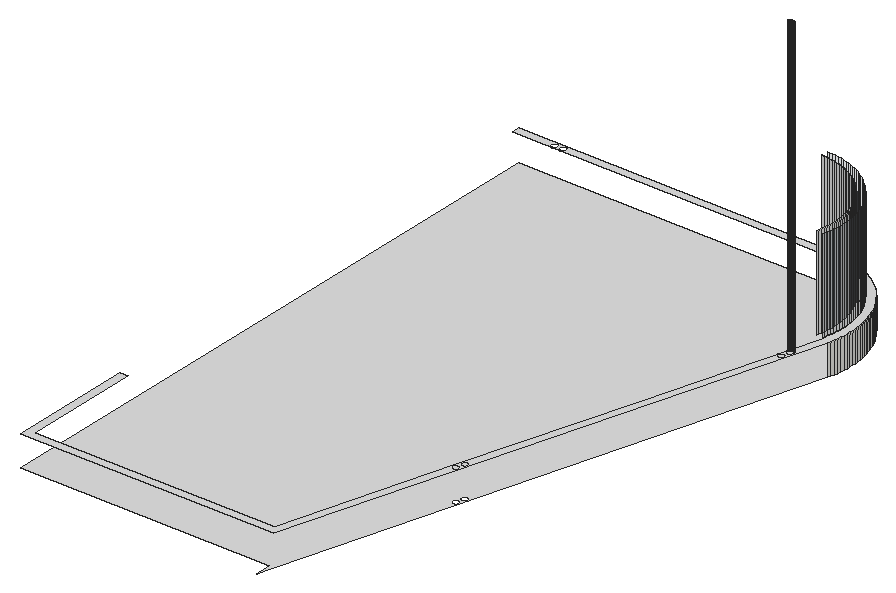
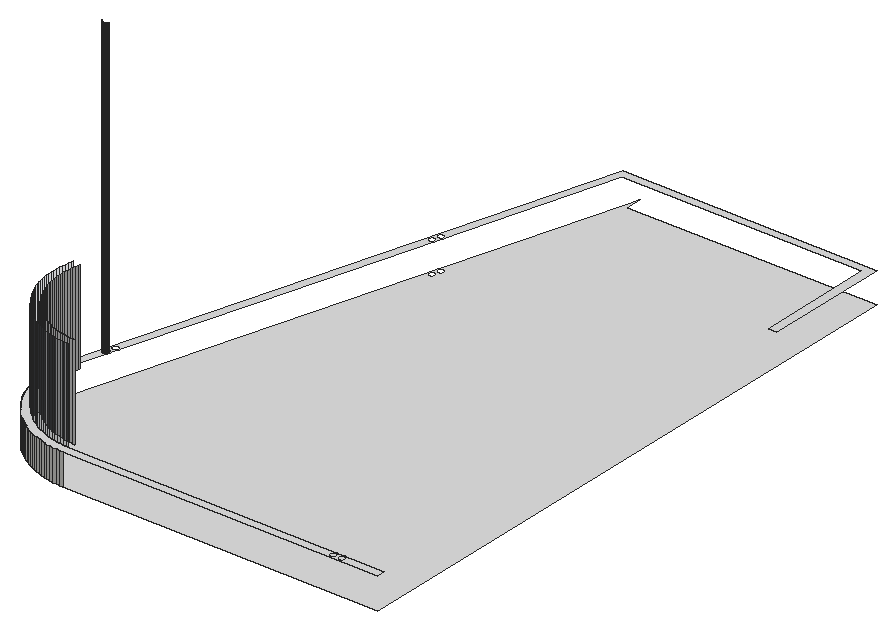
# SketchUp Ruby script. Lengths in inches.
U = 1.inch
M = Sketchup.active_model
def pt(a) = Geom::Point3d.new(a.map { |v| v * U })
def face(e, loops, mat)
  f = e.add_face(loops[0].map { |a| pt(a) })
  loops[1..].each { |l| e.add_face(l.map { |a| pt(a) }).erase! }
  f.material = f.back_material = mat if mat
  f
end
# faces: each face lists its corners as indices into pts; further lists are holes
def faces(e, pts, list, mat = nil) = list.each { |f| face(e, (f[0].is_a?(Array) ? f : [f]).map { |l| l.map { |i| pts[i] } }, mat) }
# xy, xz, yz: faces in a plane at the given z, y or x. An outline is a flat list of corners, or four numbers for a rectangle; further outlines are holes
def ring(l) = l.size == 4 ? [[l[0], l[1]], [l[2], l[1]], [l[2], l[3]], [l[0], l[3]]] : l.each_slice(2).to_a
def flat(e, list, mat, &to3) = list.each { |f| face(e, (f[0].is_a?(Array) ? f : [f]).map { |l| ring(l).map { |u, v| to3.(u, v) } }, mat) }
def xy(e, z, list, mat = nil) = flat(e, list, mat) { |x, y| [x, y, z] }
def xz(e, y, list, mat = nil) = flat(e, list, mat) { |x, z| [x, y, z] }
def yz(e, x, list, mat = nil) = flat(e, list, mat) { |y, z| [x, y, z] }
def lines(e, pts, list) = list.each { |a, b| e.add_line(pt(pts[a]), pt(pts[b])) }
# prism: a flat outline (further loops are holes) pulled along v
def prism(e, loops, v, mat = nil)
  f = face(e, loops, mat); d = Geom::Vector3d.new(v.map { |x| x * U })
  f.pushpull(f.normal.samedirection?(d) ? d.length : -d.length)
end
def box(e, o, s, mat = nil) = prism(e, [[o, [o[0] + s[0], o[1], o[2]], [o[0] + s[0], o[1] + s[1], o[2]], [o[0], o[1] + s[1], o[2]]]], [0, 0, s[2]], mat)
def at(x, y, z, deg = 0) = Geom::Transformation.translation(pt([x, y, z])) * Geom::Transformation.rotation(ORIGIN, Z_AXIS, deg.degrees)
def axes(o, x, y, z) = Geom::Transformation.new([*x, 0, *y, 0, *z, 0, *pt(o).to_a, 1])
def part(name) = M.definitions.add(name)
# library, detail: a bought-in or finely detailed component or shape, given as its bounding box
def library(name, o, s) = part(name).tap { |d| box(d.entities, o, s) }
def detail(e, o, s) = box(e.add_group.entities, o, s)
def put(e, d, t, mat = nil) = e.add_instance(d, t).tap { |i| i.material = mat if mat }
def group(e, t, mat = nil) = e.add_group.tap { |g| g.transformation = t; g.material = mat if mat }.entities
root = M.entities
M.materials.add("Glass_Basic_01").color = [105, 113, 122]
M.materials["Glass_Basic_01"].alpha = 0.25
M.materials.add("M01_Silver_Fog").color = [224, 224, 224]
xy(root,510,[[[306,234,306,240,210,240,210,480,331.55,480,332.69,479.96,334.03,479.87,335.37,479.72,336.7,479.52,338.02,479.28,339.33,478.98,340.63,478.63,341.92,478.23,343.1875,477.79,344.44,477.29,345.67,476.75,346.88,476.16,348.07,475.53,349.23,474.85,350.37,474.13,351.47,473.37,352.55,472.5625,353.6,471.72,354.61,470.83,355.59,469.91,356.53,468.95,357.39,468,357.4375,467.95,358.3,466.92,359.13,465.86,359.92,464.77,360.66,463.65,360.69,463.59,361.36,462.5,362.02,461.33,362.63,460.13,363.2,458.91,363.71,457.67,364.18,456.41,364.61,455.13,364.98,453.84,365.3,452.53,365.58,451.21,365.8,449.89,365.98,448.55,366.1,447.21,366.17,445.87,366.1875,444.52,366.16,443.18,366.07,441.84,365.94,440.5,365.76,439.16,365.52,437.84,365.24,436.52,364.95,435.42,307.76,240],[325.27,304.17,325.44,304.17,325.53,304.1875,325.62,304.2,325.7,304.22,325.79,304.25,325.87,304.28,326.03,304.36,326.24,304.51,326.3,304.57,326.42,304.71,326.52,304.85,326.5625,304.93,326.6,305.01,326.66,305.17,326.68,305.26,326.7,305.34,326.72,305.52,326.72,305.61,326.71,305.69,326.7,305.78,326.6875,305.87,326.67,305.95,326.64,306.04,326.61,306.12,326.53,306.28,326.43,306.42,326.375,306.49,326.31,306.55,326.25,306.61,326.18,306.67,326.04,306.77,325.96,306.8125,325.88,306.85,325.72,306.91,325.63,306.93,325.55,306.95,325.37,306.97,325.28,306.97,325.2,306.96,325.11,306.95,325.02,306.9375,324.9375,306.92,324.85,306.89,324.77,306.86,324.61,306.78,324.47,306.68,324.4,306.625,324.33,306.56,324.27,306.5,324.12,306.29,324,306.05,323.98,305.97,323.96,305.88,323.9375,305.8,323.93,305.71,323.92,305.62,323.92,305.53,323.93,305.44,323.9375,305.36,323.95,305.27,323.97,305.1875,324,305.1,324.03,305.02,324.11,304.86,324.26,304.65,324.32,304.58,324.39,304.52,324.6,304.37,324.84,304.25,324.92,304.23,325.01,304.2,325.09,304.1875,325.18,304.18],[326.2,307.35,326.375,307.35,326.46,307.36,326.55,307.38,326.63,307.4,326.72,307.43,326.8,307.46,326.96,307.54,327.17,307.69,327.3,307.82,327.35,307.88,327.4,307.96,327.45,308.03,327.49,308.11,327.53,308.1875,327.56,308.27,327.59,308.35,327.61,308.4375,327.63,308.52,327.65,308.7,327.65,308.79,327.63,308.96,327.62,309.05,327.6,309.13,327.57,309.22,327.54,309.3,327.46,309.46,327.31,309.67,327.25,309.73,327.11,309.85,326.97,309.95,326.89,309.99,326.8125,310.03,326.73,310.0625,326.65,310.09,326.5625,310.11,326.48,310.13,326.3,310.15,326.21,310.15,326.04,310.13,325.95,310.12,325.87,310.1,325.78,310.07,325.7,310.04,325.54,309.96,325.4,309.86,325.33,309.8,325.27,309.74,325.2,309.68,325.05,309.47,325.01,309.39,324.97,309.3125,324.9375,309.23,324.91,309.15,324.89,309.0625,324.87,308.98,324.85,308.8,324.85,308.71,324.87,308.54,324.88,308.45,324.9,308.37,324.93,308.28,324.96,308.2,325.04,308.04,325.14,307.9,325.26,307.76,325.32,307.7,325.53,307.55,325.61,307.5,325.6875,307.47,325.77,307.43,325.85,307.41,325.9375,307.38,326.02,307.37]]],"M01_Silver_Fog")
xy(root,522,[[[210,240,307.76,240,364.95,435.42,365.24,436.52,365.52,437.84,365.76,439.16,365.94,440.5,366.07,441.84,366.16,443.18,366.1875,444.52,366.17,445.87,366.1,447.21,365.98,448.55,365.8,449.89,365.58,451.21,365.3,452.53,364.98,453.84,364.61,455.13,364.18,456.41,363.71,457.67,363.2,458.91,362.63,460.13,362.02,461.33,361.36,462.5,360.69,463.59,360.66,463.65,359.92,464.77,359.13,465.86,358.3,466.92,357.4375,467.95,357.39,468,356.53,468.95,355.59,469.91,354.61,470.83,353.6,471.72,352.55,472.5625,351.47,473.37,350.37,474.13,349.23,474.85,348.07,475.53,346.88,476.16,345.67,476.75,344.44,477.29,343.1875,477.79,341.92,478.23,340.63,478.63,339.33,478.98,338.02,479.28,336.7,479.52,335.37,479.72,334.03,479.87,332.69,479.96,331.55,480,210,480,210,477,331.5,477,332.53,476.97,333.76,476.88,334.99,476.74,336.2,476.5625,337.41,476.34,338.61,476.0625,339.8,475.75,340.98,475.38,342.14,474.97,343.29,474.52,344.41,474.03,345.52,473.49,346.61,472.91,347.67,472.29,348.71,471.63,349.72,470.93,350.71,470.19,351.67,469.42,352.59,468.61,353.49,467.76,354.35,466.89,355.17,465.98,355.18,465.98,355.97,465.03,356.73,464.0625,357.45,463.0625,358.13,462.04,358.13,462.03,358.77,460.99,359.37,459.91,359.93,458.82,360.45,457.7,360.92,456.5625,361.35,455.41,361.74,454.24,362.08,453.06,362.38,451.86,362.63,450.66,362.83,449.44,362.99,448.22,363.1,447,363.17,445.77,363.1875,444.54,363.16,443.31,363.08,442.08,362.96,440.85,362.79,439.63,362.58,438.42,362.32,437.22,362.06,436.22,343.2,371.78,324.34,307.35,305.51,243,213,243,213,288,210,288],[358.91,418.8,358.82,418.81,358.73,418.8125,358.65,418.83,358.5625,418.85,358.48,418.87,358.39,418.9,358.3125,418.9375,358.24,418.98,358.16,419.02,358.09,419.07,357.95,419.18,357.89,419.24,357.83,419.31,357.73,419.45,357.68,419.53,357.64,419.61,357.61,419.6875,357.58,419.77,357.55,419.85,357.54,419.94,357.52,420.03,357.51,420.11,357.51,420.29,357.52,420.38,357.54,420.46,357.55,420.55,357.58,420.64,357.64,420.8,357.68,420.88,357.73,420.95,357.78,421.03,357.83,421.09,357.89,421.16,357.95,421.22,358.09,421.34,358.16,421.38,358.24,421.43,358.3125,421.47,358.39,421.5,358.48,421.53,358.5625,421.56,358.65,421.58,358.73,421.59,358.82,421.6,359,421.6,359.09,421.59,359.17,421.58,359.26,421.56,359.34,421.53,359.43,421.5,359.51,421.47,359.58,421.43,359.66,421.38,359.73,421.34,359.87,421.22,359.93,421.16,359.99,421.09,360.04,421.03,360.09,420.95,360.14,420.88,360.18,420.8,360.24,420.64,360.27,420.55,360.29,420.46,360.3,420.38,360.31,420.29,360.31,420.11,360.3,420.03,360.29,419.94,360.27,419.85,360.24,419.77,360.21,419.6875,360.18,419.61,360.14,419.53,360.09,419.45,359.99,419.31,359.93,419.24,359.87,419.18,359.73,419.07,359.66,419.02,359.58,418.98,359.51,418.9375,359.43,418.9,359.34,418.87,359.26,418.85,359.17,418.83,359.09,418.8125,359,418.81],[359.74,421.95,359.66,421.96,359.57,421.97,359.48,421.99,359.32,422.05,359.23,422.08,359.16,422.12,359.08,422.17,359.01,422.21,358.9375,422.27,358.87,422.33,358.75,422.45,358.7,422.52,358.65,422.6,358.6,422.67,358.5625,422.75,358.53,422.83,358.5,422.91,358.47,423,358.46,423.08,358.44,423.17,358.43,423.26,358.43,423.44,358.44,423.52,358.46,423.61,358.47,423.7,358.53,423.86,358.5625,423.94,358.6,424.02,358.65,424.1,358.75,424.24,358.81,424.31,358.87,424.37,358.9375,424.43,359.01,424.48,359.08,424.53,359.16,424.57,359.23,424.61,359.32,424.65,359.4,424.68,359.48,424.7,359.66,424.74,359.74,424.74,359.83,424.75,359.92,424.74,360.01,424.74,360.09,424.72,360.18,424.7,360.26,424.68,360.35,424.65,360.51,424.57,360.58,424.53,360.72,424.43,360.79,424.37,360.85,424.31,360.91,424.24,361.01,424.1,361.06,424.02,361.1,423.94,361.16,423.78,361.1875,423.7,361.21,423.61,361.22,423.52,361.23,423.44,361.23,423.26,361.21,423.08,361.1875,423,361.16,422.91,361.1,422.75,361.06,422.67,361.01,422.6,360.96,422.52,360.91,422.45,360.79,422.33,360.65,422.21,360.58,422.17,360.51,422.12,360.43,422.08,360.35,422.05,360.26,422.02,360.18,421.99,360.09,421.97,360.01,421.96,359.92,421.95],[228.34,477.03,228.25,477.04,228.17,477.06,228.08,477.08,228,477.11,227.91,477.14,227.84,477.18,227.76,477.22,227.68,477.27,227.54,477.37,227.48,477.43,227.42,477.5,227.36,477.56,227.3125,477.64,227.26,477.71,227.18,477.87,227.15,477.95,227.125,478.03,227.1,478.12,227.09,478.2,227.07,478.29,227.07,478.55,227.08,478.64,227.1,478.73,227.12,478.8125,227.15,478.9,227.18,478.98,227.22,479.06,227.26,479.13,227.31,479.21,227.41,479.35,227.47,479.41,227.61,479.53,227.75,479.63,227.91,479.71,228.07,479.77,228.16,479.79,228.24,479.81,228.33,479.82,228.42,479.82,228.51,479.83,228.59,479.82,228.68,479.81,228.77,479.79,228.85,479.77,228.9375,479.74,229.02,479.71,229.1,479.68,229.18,479.63,229.25,479.59,229.32,479.53,229.39,479.48,229.45,479.42,229.51,479.35,229.57,479.29,229.62,479.22,229.67,479.14,229.71,479.07,229.75,478.99,229.78,478.9,229.81,478.82,229.83,478.74,229.85,478.65,229.86,478.5625,229.87,478.47,229.87,478.39,229.85,478.21,229.83,478.125,229.8125,478.04,229.79,477.96,229.75,477.875,229.72,477.79,229.67,477.72,229.63,477.64,229.58,477.57,229.52,477.5,229.46,477.4375,229.4,477.38,229.33,477.32,229.26,477.27,229.18,477.22,229.11,477.18,229.03,477.14,228.95,477.11,228.86,477.08,228.78,477.06,228.69,477.04,228.6,477.03],[225.03,477.03,224.94,477.04,224.85,477.06,224.77,477.08,224.68,477.11,224.6,477.14,224.52,477.18,224.45,477.22,224.37,477.27,224.23,477.37,224.17,477.43,224.11,477.5,224.05,477.56,224,477.64,223.95,477.71,223.87,477.87,223.84,477.95,223.8125,478.03,223.77,478.2,223.76,478.29,223.76,478.55,223.77,478.64,223.79,478.73,223.81,478.8125,223.84,478.9,223.87,478.98,223.91,479.06,223.95,479.13,223.99,479.21,224.05,479.28,224.1,479.35,224.16,479.41,224.23,479.47,224.29,479.53,224.36,479.58,224.4375,479.63,224.52,479.67,224.6,479.71,224.76,479.77,224.85,479.79,224.93,479.81,225.02,479.82,225.11,479.82,225.19,479.83,225.37,479.81,225.46,479.79,225.54,479.77,225.71,479.71,225.79,479.68,225.86,479.63,225.9375,479.59,226.01,479.53,226.08,479.48,226.14,479.42,226.2,479.35,226.26,479.29,226.3125,479.22,226.36,479.14,226.4,479.07,226.4375,478.99,226.47,478.9,226.5,478.82,226.52,478.74,226.54,478.65,226.55,478.5625,226.55,478.3,226.54,478.21,226.5,478.04,226.47,477.96,226.44,477.875,226.4,477.79,226.36,477.72,226.32,477.64,226.26,477.57,226.21,477.5,226.15,477.4375,226.08,477.38,226.02,477.32,225.95,477.27,225.87,477.22,225.71,477.14,225.55,477.08,225.46,477.06,225.38,477.04,225.29,477.03],[325.27,304.17,325.18,304.18,325.09,304.1875,325.01,304.2,324.92,304.23,324.84,304.25,324.6,304.37,324.39,304.52,324.32,304.58,324.26,304.65,324.11,304.86,324.03,305.02,324,305.1,323.97,305.1875,323.95,305.27,323.9375,305.36,323.93,305.44,323.92,305.53,323.92,305.62,323.93,305.71,323.9375,305.8,323.96,305.88,323.98,305.97,324,306.05,324.12,306.29,324.27,306.5,324.33,306.56,324.4,306.625,324.47,306.68,324.61,306.78,324.77,306.86,324.85,306.89,324.9375,306.92,325.02,306.9375,325.11,306.95,325.2,306.96,325.28,306.97,325.37,306.97,325.55,306.95,325.63,306.93,325.72,306.91,325.88,306.85,325.96,306.8125,326.04,306.77,326.18,306.67,326.25,306.61,326.31,306.55,326.375,306.49,326.43,306.42,326.53,306.28,326.61,306.12,326.64,306.04,326.67,305.95,326.6875,305.87,326.7,305.78,326.71,305.69,326.72,305.61,326.72,305.52,326.7,305.34,326.68,305.26,326.66,305.17,326.6,305.01,326.5625,304.93,326.52,304.85,326.42,304.71,326.3,304.57,326.24,304.51,326.03,304.36,325.87,304.28,325.79,304.25,325.7,304.22,325.62,304.2,325.53,304.1875,325.44,304.17],[326.2,307.35,326.02,307.37,325.9375,307.38,325.85,307.41,325.77,307.43,325.6875,307.47,325.61,307.5,325.53,307.55,325.32,307.7,325.26,307.76,325.14,307.9,325.04,308.04,324.96,308.2,324.93,308.28,324.9,308.37,324.88,308.45,324.87,308.54,324.85,308.71,324.85,308.8,324.87,308.98,324.89,309.0625,324.91,309.15,324.9375,309.23,324.97,309.3125,325.01,309.39,325.05,309.47,325.2,309.68,325.27,309.74,325.33,309.8,325.4,309.86,325.54,309.96,325.7,310.04,325.78,310.07,325.87,310.1,325.95,310.12,326.04,310.13,326.21,310.15,326.3,310.15,326.48,310.13,326.5625,310.11,326.65,310.09,326.73,310.0625,326.8125,310.03,326.89,309.99,326.97,309.95,327.11,309.85,327.25,309.73,327.31,309.67,327.46,309.46,327.54,309.3,327.57,309.22,327.6,309.13,327.62,309.05,327.63,308.96,327.65,308.79,327.65,308.7,327.63,308.52,327.61,308.4375,327.59,308.35,327.56,308.27,327.53,308.1875,327.49,308.11,327.45,308.03,327.4,307.96,327.35,307.88,327.3,307.82,327.17,307.69,326.96,307.54,326.8,307.46,326.72,307.43,326.63,307.4,326.55,307.38,326.46,307.36,326.375,307.35]]],"M01_Silver_Fog")
xz(root,424.74,[[359.66,522,359.74,636],[359.92,522,360.01,636]],"M01_Silver_Fog")
xz(root,465.98,[[355.17,522,355.18,558]],"Glass_Basic_01")
yz(root,358.13,[[462.03,522,462.04,558]],"Glass_Basic_01")
p = [[365.24,436.52,522],[364.95,435.42,522],[364.95,435.42,510],[365.24,436.52,510],[365.52,437.84,522],[365.52,437.84,510],
  [365.76,439.16,522],[365.76,439.16,510],[365.94,440.5,522],[365.94,440.5,510],[366.07,441.84,522],[366.07,441.84,510],
  [366.16,443.18,522],[366.16,443.18,510],[366.1875,444.52,522],[366.1875,444.52,510],[366.17,445.87,522],[366.17,445.87,510],
  [366.1,447.21,522],[366.1,447.21,510],[365.98,448.55,522],[365.98,448.55,510],[365.8,449.89,522],[365.8,449.89,510],
  [365.58,451.21,522],[365.58,451.21,510],[365.3,452.53,522],[365.3,452.53,510],[364.98,453.84,522],[364.98,453.84,510],
  [364.61,455.13,522],[364.61,455.13,510],[364.18,456.41,522],[364.18,456.41,510],[363.71,457.67,522],[363.71,457.67,510],
  [363.2,458.91,522],[363.2,458.91,510],[362.63,460.13,522],[362.63,460.13,510],[362.02,461.33,522],[362.02,461.33,510],
  [361.36,462.5,522],[361.36,462.5,510],[360.69,463.59,522],[360.69,463.59,510],[359.92,464.77,522],[360.66,463.65,522],
  [360.66,463.65,510],[359.92,464.77,510],[359.13,465.86,522],[359.13,465.86,510],[358.3,466.92,522],[358.3,466.92,510],
  [357.4375,467.95,522],[357.4375,467.95,510],[356.53,468.95,522],[357.39,468,522],[357.39,468,510],[356.53,468.95,510],
  [355.59,469.91,522],[355.59,469.91,510],[354.61,470.83,522],[354.61,470.83,510],[353.6,471.72,522],[353.6,471.72,510],
  [352.55,472.5625,522],[352.55,472.5625,510],[351.47,473.37,522],[351.47,473.37,510],[350.37,474.13,522],[350.37,474.13,510],
  [349.23,474.85,522],[349.23,474.85,510],[348.07,475.53,522],[348.07,475.53,510],[346.88,476.16,522],[346.88,476.16,510],
  [345.67,476.75,522],[345.67,476.75,510],[344.44,477.29,522],[344.44,477.29,510],[343.1875,477.79,522],[343.1875,477.79,510],
  [341.92,478.23,522],[341.92,478.23,510],[340.63,478.63,522],[340.63,478.63,510],[339.33,478.98,522],[339.33,478.98,510],
  [338.02,479.28,522],[338.02,479.28,510],[336.7,479.52,522],[336.7,479.52,510],[335.37,479.72,522],[335.37,479.72,510],
  [334.03,479.87,522],[334.03,479.87,510],[332.69,479.96,522],[332.69,479.96,510],[331.55,480,522],[331.55,480,510],
  [358.6,424.02,522],[358.5625,423.94,522],[358.5625,423.94,636],[358.6,424.02,636],[361.1,423.94,522],[361.06,424.02,522],
  [361.06,424.02,636],[361.1,423.94,636],[358.65,424.1,522],[358.65,424.1,636],[361.01,424.1,522],[361.01,424.1,636],
  [358.7,424.17,522],[358.7,424.17,636],[360.96,424.17,522],[360.96,424.17,636],[358.75,424.24,522],[358.75,424.24,636],
  [358.81,424.31,522],[358.81,424.31,636],[360.91,424.24,522],[360.91,424.24,636],[360.85,424.31,522],[360.85,424.31,636],
  [358.87,424.37,522],[358.87,424.37,636],[360.79,424.37,522],[360.79,424.37,636],[358.9375,424.43,522],[358.9375,424.43,636],
  [359.01,424.48,522],[359.01,424.48,636],[360.72,424.43,522],[360.72,424.43,636],[360.65,424.48,522],[360.65,424.48,636],
  [359.08,424.53,522],[359.08,424.53,636],[359.16,424.57,522],[359.16,424.57,636],[360.58,424.53,522],[360.51,424.57,522],
  [360.51,424.57,636],[360.58,424.53,636],[359.23,424.61,522],[359.23,424.61,636],[359.32,424.65,522],[359.32,424.65,636],
  [359.4,424.68,522],[359.4,424.68,636],[360.43,424.61,522],[360.35,424.65,522],[360.35,424.65,636],[360.43,424.61,636],
  [360.26,424.68,522],[360.26,424.68,636],[359.48,424.7,522],[359.48,424.7,636],[359.57,424.72,522],[359.57,424.72,636],
  [359.66,424.74,522],[359.66,424.74,636],[359.83,424.75,522],[359.74,424.74,522],[359.74,424.74,636],[359.83,424.75,636],
  [359.92,424.74,522],[359.92,424.74,636],[360.09,424.72,522],[360.01,424.74,522],[360.01,424.74,636],[360.09,424.72,636],
  [360.18,424.7,522],[360.18,424.7,636],[362.06,436.22,522],[362.32,437.22,522],[362.32,437.22,558],[362.06,436.22,558],
  [359.4,437.91,522],[359.17,437.01,522],[359.17,437.01,558],[359.4,437.91,558],[362.58,438.42,522],[362.58,438.42,558],
  [359.63,439,522],[359.63,439,558],[362.79,439.63,522],[362.79,439.63,558],[359.83,440.1,522],[359.83,440.1,558],
  [362.96,440.85,522],[362.96,440.85,558],[359.98,441.21,522],[359.98,441.21,558],[363.08,442.08,522],[363.08,442.08,558],
  [360.09,442.32,522],[360.09,442.32,558],[363.16,443.31,522],[363.16,443.31,558],[360.16,443.43,522],[360.16,443.43,558],
  [363.1875,444.54,522],[363.1875,444.54,558],[360.1875,444.55,522],[360.1875,444.55,558],[360.17,445.67,522],[360.17,445.67,558],
  [363.17,445.77,522],[363.17,445.77,558],[360.11,446.78,522],[360.11,446.78,558],[363.1,447,522],[363.1,447,558],
  [360.01,447.89,522],[360.01,447.89,558],[362.99,448.22,522],[362.99,448.22,558],[359.87,449,522],[359.87,449,558],
  [362.83,449.44,522],[362.83,449.44,558],[359.68,450.1,522],[359.68,450.1,558],[362.63,450.66,522],[362.63,450.66,558],
  [359.45,451.2,522],[359.45,451.2,558],[362.38,451.86,522],[362.38,451.86,558],[359.18,452.28,522],[359.18,452.28,558],
  [362.08,453.06,522],[362.08,453.06,558],[358.875,453.35,522],[358.875,453.35,558],[361.74,454.24,522],[361.74,454.24,558],
  [358.52,454.41,522],[358.52,454.41,558],[361.35,455.41,522],[361.35,455.41,558],[358.13,455.46,522],[358.13,455.46,558],
  [360.92,456.5625,522],[360.92,456.5625,558],[357.7,456.49,522],[357.7,456.49,558],[357.23,457.5,522],[357.23,457.5,558],
  [360.45,457.7,522],[360.45,457.7,558],[356.73,458.5,522],[356.73,458.5,558],[359.93,458.82,522],[359.93,458.82,558],
  [356.18,459.47,522],[356.18,459.47,558],[359.37,459.91,522],[359.37,459.91,558],[355.6,460.43,522],[355.6,460.43,558],
  [358.77,460.99,522],[358.77,460.99,558],[354.98,461.36,522],[354.98,461.36,558],[358.13,462.03,522],[358.13,462.03,558],
  [354.33,462.26,522],[354.33,462.26,558],[358.13,462.04,522],[357.45,463.0625,522],[357.45,463.0625,558],[358.13,462.04,558],
  [353.64,463.14,522],[353.64,463.14,558],[352.92,464,522],[352.92,464,558],[356.73,464.0625,522],[356.73,464.0625,558],
  [352.17,464.83,522],[352.17,464.83,558],[355.97,465.03,522],[355.97,465.03,558],[351.39,465.62,522],[351.39,465.62,558],
  [355.18,465.98,522],[355.18,465.98,558],[350.58,466.39,522],[350.58,466.39,558],[355.17,465.98,522],[354.35,466.89,522],
  [354.35,466.89,558],[355.17,465.98,558],[349.74,467.125,522],[349.74,467.125,558],[353.49,467.76,522],[353.49,467.76,558],
  [348.87,467.83,522],[348.87,467.83,558],[347.97,468.5,522],[347.97,468.5,558],[352.59,468.61,522],[352.59,468.61,558],
  [347.05,469.13,522],[347.05,469.13,558],[351.67,469.42,522],[351.67,469.42,558],[346.11,469.73,522],[346.11,469.73,558],
  [350.71,470.19,522],[350.71,470.19,558],[345.15,470.29,522],[345.15,470.29,558],[349.72,470.93,522],[349.72,470.93,558],
  [344.16,470.82,522],[344.16,470.82,558],[343.16,471.3,522],[343.16,471.3,558],[348.71,471.63,522],[348.71,471.63,558],
  [342.13,471.75,522],[342.13,471.75,558],[347.67,472.29,522],[347.67,472.29,558],[341.09,472.16,522],[341.09,472.16,558],
  [340.04,472.53,522],[340.04,472.53,558],[346.61,472.91,522],[346.61,472.91,558],[338.97,472.86,522],[338.97,472.86,558],
  [337.89,473.15,522],[337.89,473.15,558],[345.52,473.49,522],[345.52,473.49,558],[336.8,473.4,522],[336.8,473.4,558],
  [335.71,473.6,522],[335.71,473.6,558],[344.41,474.03,522],[344.41,474.03,558],[334.6,473.77,522],[334.6,473.77,558],
  [333.49,473.89,522],[333.49,473.89,558],[332.38,473.97,522],[332.38,473.97,558],[331.45,474,522],[331.45,474,558],
  [343.29,474.52,522],[343.29,474.52,558],[342.14,474.97,522],[342.14,474.97,558],[340.98,475.38,522],[340.98,475.38,558],
  [339.8,475.75,522],[339.8,475.75,558],[338.61,476.0625,522],[338.61,476.0625,558],[337.41,476.34,522],[337.41,476.34,558],
  [336.2,476.5625,522],[336.2,476.5625,558],[334.99,476.74,522],[334.99,476.74,558],[333.76,476.88,522],[333.76,476.88,558],
  [332.53,476.97,522],[332.53,476.97,558],[331.5,477,522],[331.5,477,558]]
faces(root,p,[[0,1,2,3],[4,0,3,5],[6,4,5,7],[8,6,7,9],[10,8,9,11],[12,10,11,13],[14,12,13,15],[16,14,15,17],
  [18,16,17,19],[20,18,19,21],[22,20,21,23],[24,22,23,25],[26,24,25,27],[28,26,27,29],[30,28,29,31],[32,30,31,33],
  [34,32,33,35],[36,34,35,37],[38,36,37,39],[40,38,39,41],[42,40,41,43],[44,42,43,45],[46,47,48,49],[47,44,45,48],
  [50,46,49,51],[52,50,51,53],[54,52,53,55],[56,57,58,59],[57,54,55,58],[60,56,59,61],[62,60,61,63],[64,62,63,65],
  [66,64,65,67],[68,66,67,69],[70,68,69,71],[72,70,71,73],[74,72,73,75],[76,74,75,77],[78,76,77,79],[80,78,79,81],
  [82,80,81,83],[84,82,83,85],[86,84,85,87],[88,86,87,89],[90,88,89,91],[92,90,91,93],[94,92,93,95],[96,94,95,97],
  [98,96,97,99],[100,98,99,101]])
faces(root,p,[[102,103,104,105],[106,107,108,109],[110,102,105,111],[107,112,113,108],[114,110,111,115],[112,116,117,113],[118,114,115,119],[120,118,119,121],
  [116,122,123,117],[122,124,125,123],[126,120,121,127],[124,128,129,125],[130,126,127,131],[132,130,131,133],[128,134,135,129],[134,136,137,135],
  [138,132,133,139],[140,138,139,141],[142,143,144,145],[136,142,145,137],[146,140,141,147],[148,146,147,149],[150,148,149,151],[152,153,154,155],
  [153,156,157,154],[143,152,155,144],[158,150,151,159],[160,158,159,161],[162,160,161,163],[164,165,166,167],[168,164,167,169],[170,171,172,173],
  [174,170,173,175],[156,174,175,157],[180,181,182,183],[186,180,183,187],[190,186,187,191],[194,190,191,195],[198,194,195,199],[202,198,199,203],
  [206,202,203,207],[208,206,207,209],[212,208,209,213],[216,212,213,217],[220,216,217,221],[224,220,221,225],[228,224,225,229],[232,228,229,233],
  [236,232,233,237],[240,236,237,241],[244,240,241,245],[248,244,245,249],[250,248,249,251],[254,250,251,255],[258,254,255,259],[262,258,259,263],
  [266,262,263,267],[270,266,267,271],[276,270,271,277],[278,276,277,279],[282,278,279,283],[286,282,283,287],[290,286,287,291],[296,290,291,297],
  [300,296,297,301],[302,300,301,303],[306,302,303,307],[310,306,307,311],[314,310,311,315],[318,314,315,319],[320,318,319,321],[324,320,321,325],
  [328,324,325,329],[330,328,329,331],[334,330,331,335],[336,334,335,337],[340,336,337,341],[342,340,341,343],[346,342,343,347],[348,346,347,349],
  [350,348,349,351],[352,350,351,353]],"M01_Silver_Fog")
faces(root,p,[[176,177,178,179],[177,184,185,178],[184,188,189,185],[188,192,193,189],[192,196,197,193],[196,200,201,197],[200,204,205,201],[204,210,211,205],
  [210,214,215,211],[214,218,219,215],[218,222,223,219],[222,226,227,223],[226,230,231,227],[230,234,235,231],[234,238,239,235],[238,242,243,239],
  [242,246,247,243],[246,252,253,247],[252,256,257,253],[256,260,261,257],[260,264,265,261],[264,268,269,265],[272,273,274,275],[273,280,281,274],
  [280,284,285,281],[284,288,289,285],[292,293,294,295],[293,298,299,294],[298,304,305,299],[304,308,309,305],[308,312,313,309],[312,316,317,313],
  [316,322,323,317],[322,326,327,323],[326,332,333,327],[332,338,339,333],[338,344,345,339],[344,354,355,345],[354,356,357,355],[356,358,359,357],
  [358,360,361,359],[360,362,363,361],[362,364,365,363],[364,366,367,365],[366,368,369,367],[368,370,371,369],[370,372,373,371],[372,374,375,373]],"Glass_Basic_01")
